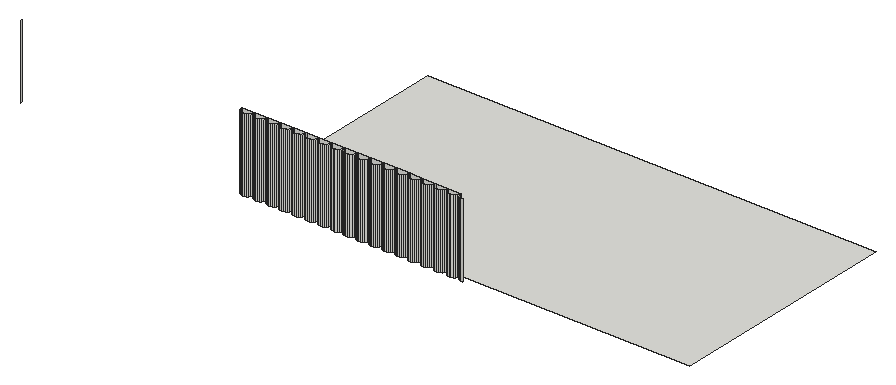
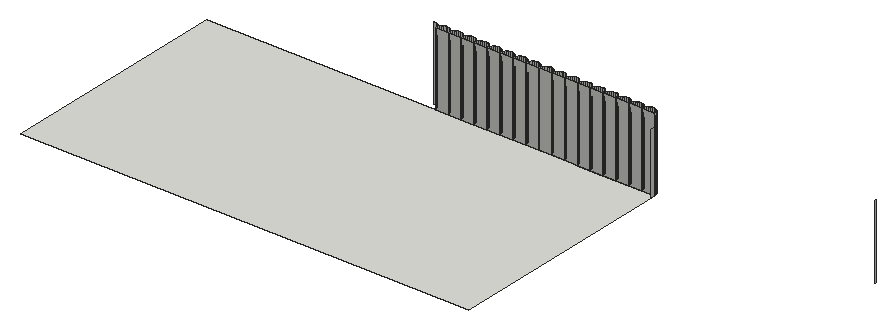
# SketchUp Ruby script. Lengths in inches.
U = 1.inch
M = Sketchup.active_model
def pt(a) = Geom::Point3d.new(a.map { |v| v * U })
def face(e, loops, mat)
  f = e.add_face(loops[0].map { |a| pt(a) })
  loops[1..].each { |l| e.add_face(l.map { |a| pt(a) }).erase! }
  f.material = f.back_material = mat if mat
  f
end
# faces: each face lists its corners as indices into pts; further lists are holes
def faces(e, pts, list, mat = nil) = list.each { |f| face(e, (f[0].is_a?(Array) ? f : [f]).map { |l| l.map { |i| pts[i] } }, mat) }
# xy, xz, yz: faces in a plane at the given z, y or x. An outline is a flat list of corners, or four numbers for a rectangle; further outlines are holes
def ring(l) = l.size == 4 ? [[l[0], l[1]], [l[2], l[1]], [l[2], l[3]], [l[0], l[3]]] : l.each_slice(2).to_a
def flat(e, list, mat, &to3) = list.each { |f| face(e, (f[0].is_a?(Array) ? f : [f]).map { |l| ring(l).map { |u, v| to3.(u, v) } }, mat) }
def xy(e, z, list, mat = nil) = flat(e, list, mat) { |x, y| [x, y, z] }
def xz(e, y, list, mat = nil) = flat(e, list, mat) { |x, z| [x, y, z] }
def yz(e, x, list, mat = nil) = flat(e, list, mat) { |y, z| [x, y, z] }
def lines(e, pts, list) = list.each { |a, b| e.add_line(pt(pts[a]), pt(pts[b])) }
# prism: a flat outline (further loops are holes) pulled along v
def prism(e, loops, v, mat = nil)
  f = face(e, loops, mat); d = Geom::Vector3d.new(v.map { |x| x * U })
  f.pushpull(f.normal.samedirection?(d) ? d.length : -d.length)
end
def box(e, o, s, mat = nil) = prism(e, [[o, [o[0] + s[0], o[1], o[2]], [o[0] + s[0], o[1] + s[1], o[2]], [o[0], o[1] + s[1], o[2]]]], [0, 0, s[2]], mat)
def at(x, y, z, deg = 0) = Geom::Transformation.translation(pt([x, y, z])) * Geom::Transformation.rotation(ORIGIN, Z_AXIS, deg.degrees)
def axes(o, x, y, z) = Geom::Transformation.new([*x, 0, *y, 0, *z, 0, *pt(o).to_a, 1])
def part(name) = M.definitions.add(name)
# library, detail: a bought-in or finely detailed component or shape, given as its bounding box
def library(name, o, s) = part(name).tap { |d| box(d.entities, o, s) }
def detail(e, o, s) = box(e.add_group.entities, o, s)
def put(e, d, t, mat = nil) = e.add_instance(d, t).tap { |i| i.material = mat if mat }
def group(e, t, mat = nil) = e.add_group.tap { |g| g.transformation = t; g.material = mat if mat }.entities
root = M.entities
xy(root,33.18,[[74.21,140.54,74.05,140.5625,73.89,140.63,73.75,140.73,73.65,140.87,73.58,141.03,73.56,141.2,74.87,141.2,74.85,141.03,74.78,140.87,74.68,140.73,74.54,140.63,74.38,140.5625],[75.53,140.54,75.36,140.5625,75.2,140.63,75.0625,140.73,74.96,140.87,74.89,141.03,74.87,141.2,76.18,141.2,76.16,141.03,76.1,140.87,75.99,140.73,75.86,140.63,75.7,140.5625],[76.84,140.54,76.67,140.5625,76.51,140.63,76.375,140.73,76.27,140.87,76.21,141.03,76.18,141.2,77.5,141.2,77.47,141.03,77.41,140.87,77.3,140.73,77.17,140.63,77.01,140.5625],[78.15,140.54,77.98,140.5625,77.82,140.63,77.6875,140.73,77.58,140.87,77.52,141.03,77.5,141.2,78.81,141.2,78.79,141.03,78.72,140.87,78.62,140.73,78.48,140.63,78.32,140.5625],[79.46,140.54,79.3,140.5625,79.14,140.63,79,140.73,78.9,140.87,78.83,141.03,78.81,141.2,80.12,141.2,80.1,141.03,80.03,140.87,79.93,140.73,79.79,140.63,79.63,140.5625],
  [80.78,140.54,80.61,140.5625,80.45,140.63,80.3125,140.73,80.21,140.87,80.14,141.03,80.12,141.2,81.43,141.2,81.41,141.03,81.35,140.87,81.24,140.73,81.11,140.63,80.95,140.5625],[82.09,140.54,81.92,140.5625,81.76,140.63,81.625,140.73,81.52,140.87,81.46,141.03,81.43,141.2,82.75,141.2,82.72,141.03,82.66,140.87,82.55,140.73,82.42,140.63,82.26,140.5625],[83.4,140.54,83.23,140.5625,83.07,140.63,82.9375,140.73,82.83,140.87,82.77,141.03,82.75,141.2,84.06,141.2,84.04,141.03,83.97,140.87,83.87,140.73,83.73,140.63,83.57,140.5625],[84.71,140.54,84.55,140.5625,84.39,140.63,84.25,140.73,84.15,140.87,84.08,141.03,84.06,141.2,85.37,141.2,85.35,141.03,85.28,140.87,85.18,140.73,85.04,140.63,84.88,140.5625],[86.03,140.54,85.86,140.5625,85.7,140.63,85.5625,140.73,85.46,140.87,85.39,141.03,85.37,141.2,86.68,141.2,86.66,141.03,86.6,140.87,86.49,140.73,86.36,140.63,86.2,140.5625],
  [87.34,140.54,87.17,140.5625,87.01,140.63,86.875,140.73,86.77,140.87,86.71,141.03,86.68,141.2,88,141.2,87.97,141.03,87.91,140.87,87.8,140.73,87.67,140.63,87.51,140.5625],[88.65,140.54,88.48,140.5625,88.32,140.63,88.1875,140.73,88.08,140.87,88.02,141.03,88,141.2,89.31,141.2,89.29,141.03,89.22,140.87,89.12,140.73,88.98,140.63,88.82,140.5625],[89.96,140.54,89.8,140.5625,89.64,140.63,89.5,140.73,89.4,140.87,89.33,141.03,89.31,141.2,90.62,141.2,90.6,141.03,90.53,140.87,90.43,140.73,90.29,140.63,90.13,140.5625],[91.28,140.54,91.11,140.5625,90.95,140.63,90.8125,140.73,90.71,140.87,90.64,141.03,90.62,141.2,91.93,141.2,91.91,141.03,91.85,140.87,91.74,140.73,91.61,140.63,91.45,140.5625],[92.59,140.54,92.42,140.5625,92.26,140.63,92.125,140.73,92.02,140.87,91.96,141.03,91.93,141.2,93.25,141.2,93.22,141.03,93.16,140.87,93.05,140.73,92.92,140.63,92.76,140.5625],
  [93.9,140.54,93.73,140.5625,93.57,140.63,93.4375,140.73,93.33,140.87,93.27,141.03,93.25,141.2,94.56,141.2,94.54,141.03,94.47,140.87,94.37,140.73,94.23,140.63,94.07,140.5625],[95.21,140.54,95.05,140.5625,94.89,140.63,94.75,140.73,94.65,140.87,94.58,141.03,94.56,141.2,95.87,141.2,95.85,141.03,95.78,140.87,95.68,140.73,95.54,140.63,95.38,140.5625],[73.56,141.2,119.1875,164.88]])
xz(root,141.2,[[73.56,33.18,74.87,40.6875],[74.87,33.18,76.18,40.6875],[76.18,33.18,77.5,40.6875],[77.5,33.18,78.81,40.6875],[78.81,33.18,80.12,40.6875],
  [80.12,33.18,81.43,40.6875],[81.43,33.18,82.75,40.6875],[82.75,33.18,84.06,40.6875],[84.06,33.18,85.37,40.6875],[85.37,33.18,86.68,40.6875],
  [86.68,33.18,88,40.6875],[88,33.18,89.31,40.6875],[89.31,33.18,90.62,40.6875],[90.62,33.18,91.93,40.6875],[91.93,33.18,93.25,40.6875],
  [93.25,33.18,94.56,40.6875],[94.56,33.18,95.87,40.6875]])
yz(root,73.56,[[141.2,33.18,141.7,39.45]])
p = [[74.05,140.5625,33.18],[74.21,140.54,33.18],[74.21,140.54,40.6875],[74.05,140.5625,40.6875],[74.38,140.5625,33.18],[74.38,140.5625,40.6875],
  [75.36,140.5625,33.18],[75.53,140.54,33.18],[75.53,140.54,40.6875],[75.36,140.5625,40.6875],[75.7,140.5625,33.18],[75.7,140.5625,40.6875],
  [76.67,140.5625,33.18],[76.84,140.54,33.18],[76.84,140.54,40.6875],[76.67,140.5625,40.6875],[77.01,140.5625,33.18],[77.01,140.5625,40.6875],
  [77.98,140.5625,33.18],[78.15,140.54,33.18],[78.15,140.54,40.6875],[77.98,140.5625,40.6875],[78.32,140.5625,33.18],[78.32,140.5625,40.6875],
  [79.3,140.5625,33.18],[79.46,140.54,33.18],[79.46,140.54,40.6875],[79.3,140.5625,40.6875],[79.63,140.5625,33.18],[79.63,140.5625,40.6875],
  [80.61,140.5625,33.18],[80.78,140.54,33.18],[80.78,140.54,40.6875],[80.61,140.5625,40.6875],[80.95,140.5625,33.18],[80.95,140.5625,40.6875],
  [81.92,140.5625,33.18],[82.09,140.54,33.18],[82.09,140.54,40.6875],[81.92,140.5625,40.6875],[82.26,140.5625,33.18],[82.26,140.5625,40.6875],
  [83.23,140.5625,33.18],[83.4,140.54,33.18],[83.4,140.54,40.6875],[83.23,140.5625,40.6875],[83.57,140.5625,33.18],[83.57,140.5625,40.6875],
  [84.55,140.5625,33.18],[84.71,140.54,33.18],[84.71,140.54,40.6875],[84.55,140.5625,40.6875],[84.88,140.5625,33.18],[84.88,140.5625,40.6875],
  [85.86,140.5625,33.18],[86.03,140.54,33.18],[86.03,140.54,40.6875],[85.86,140.5625,40.6875],[86.2,140.5625,33.18],[86.2,140.5625,40.6875],
  [87.17,140.5625,33.18],[87.34,140.54,33.18],[87.34,140.54,40.6875],[87.17,140.5625,40.6875],[87.51,140.5625,33.18],[87.51,140.5625,40.6875],
  [88.48,140.5625,33.18],[88.65,140.54,33.18],[88.65,140.54,40.6875],[88.48,140.5625,40.6875],[88.82,140.5625,33.18],[88.82,140.5625,40.6875],
  [89.8,140.5625,33.18],[89.96,140.54,33.18],[89.96,140.54,40.6875],[89.8,140.5625,40.6875],[90.13,140.5625,33.18],[90.13,140.5625,40.6875],
  [91.11,140.5625,33.18],[91.28,140.54,33.18],[91.28,140.54,40.6875],[91.11,140.5625,40.6875],[91.45,140.5625,33.18],[91.45,140.5625,40.6875],
  [92.42,140.5625,33.18],[92.59,140.54,33.18],[92.59,140.54,40.6875],[92.42,140.5625,40.6875],[92.76,140.5625,33.18],[92.76,140.5625,40.6875],
  [93.73,140.5625,33.18],[93.9,140.54,33.18],[93.9,140.54,40.6875],[93.73,140.5625,40.6875],[94.07,140.5625,33.18],[94.07,140.5625,40.6875],
  [95.05,140.5625,33.18],[95.21,140.54,33.18],[95.21,140.54,40.6875],[95.05,140.5625,40.6875],[95.38,140.5625,33.18],[95.38,140.5625,40.6875],
  [96.36,140.5625,33.18],[96.53,140.54,33.18],[96.53,140.54,40.6875],[96.36,140.5625,40.6875],[73.75,140.73,33.18],[73.89,140.63,33.18],
  [73.89,140.63,40.6875],[73.75,140.73,40.6875],[74.54,140.63,33.18],[74.54,140.63,40.6875],[74.68,140.73,33.18],[74.68,140.73,40.6875],
  [75.0625,140.73,33.18],[75.2,140.63,33.18],[75.2,140.63,40.6875],[75.0625,140.73,40.6875],[75.86,140.63,33.18],[75.86,140.63,40.6875],
  [75.99,140.73,33.18],[75.99,140.73,40.6875],[76.375,140.73,33.18],[76.51,140.63,33.18],[76.51,140.63,40.6875],[76.375,140.73,40.6875],
  [77.17,140.63,33.18],[77.17,140.63,40.6875],[77.3,140.73,33.18],[77.3,140.73,40.6875],[77.6875,140.73,33.18],[77.82,140.63,33.18],
  [77.82,140.63,40.6875],[77.6875,140.73,40.6875],[78.48,140.63,33.18],[78.48,140.63,40.6875],[78.62,140.73,33.18],[78.62,140.73,40.6875],
  [79,140.73,33.18],[79.14,140.63,33.18],[79.14,140.63,40.6875],[79,140.73,40.6875],[79.79,140.63,33.18],[79.79,140.63,40.6875],
  [79.93,140.73,33.18],[79.93,140.73,40.6875],[80.3125,140.73,33.18],[80.45,140.63,33.18],[80.45,140.63,40.6875],[80.3125,140.73,40.6875],
  [81.11,140.63,33.18],[81.11,140.63,40.6875],[81.24,140.73,33.18],[81.24,140.73,40.6875],[81.625,140.73,33.18],[81.76,140.63,33.18],
  [81.76,140.63,40.6875],[81.625,140.73,40.6875],[82.42,140.63,33.18],[82.42,140.63,40.6875],[82.55,140.73,33.18],[82.55,140.73,40.6875],
  [82.9375,140.73,33.18],[83.07,140.63,33.18],[83.07,140.63,40.6875],[82.9375,140.73,40.6875],[83.73,140.63,33.18],[83.73,140.63,40.6875],
  [83.87,140.73,33.18],[83.87,140.73,40.6875],[84.25,140.73,33.18],[84.39,140.63,33.18],[84.39,140.63,40.6875],[84.25,140.73,40.6875],
  [85.04,140.63,33.18],[85.04,140.63,40.6875],[85.18,140.73,33.18],[85.18,140.73,40.6875],[85.5625,140.73,33.18],[85.7,140.63,33.18],
  [85.7,140.63,40.6875],[85.5625,140.73,40.6875],[86.36,140.63,33.18],[86.36,140.63,40.6875],[86.49,140.73,33.18],[86.49,140.73,40.6875],
  [86.875,140.73,33.18],[87.01,140.63,33.18],[87.01,140.63,40.6875],[86.875,140.73,40.6875],[87.67,140.63,33.18],[87.67,140.63,40.6875],
  [87.8,140.73,33.18],[87.8,140.73,40.6875],[88.1875,140.73,33.18],[88.32,140.63,33.18],[88.32,140.63,40.6875],[88.1875,140.73,40.6875],
  [88.98,140.63,33.18],[88.98,140.63,40.6875],[89.12,140.73,33.18],[89.12,140.73,40.6875],[89.5,140.73,33.18],[89.64,140.63,33.18],
  [89.64,140.63,40.6875],[89.5,140.73,40.6875],[90.29,140.63,33.18],[90.29,140.63,40.6875],[90.43,140.73,33.18],[90.43,140.73,40.6875],
  [90.8125,140.73,33.18],[90.95,140.63,33.18],[90.95,140.63,40.6875],[90.8125,140.73,40.6875],[91.61,140.63,33.18],[91.61,140.63,40.6875],
  [91.74,140.73,33.18],[91.74,140.73,40.6875],[92.125,140.73,33.18],[92.26,140.63,33.18],[92.26,140.63,40.6875],[92.125,140.73,40.6875],
  [92.92,140.63,33.18],[92.92,140.63,40.6875],[93.05,140.73,33.18],[93.05,140.73,40.6875],[93.4375,140.73,33.18],[93.57,140.63,33.18],
  [93.57,140.63,40.6875],[93.4375,140.73,40.6875],[94.23,140.63,33.18],[94.23,140.63,40.6875],[94.37,140.73,33.18],[94.37,140.73,40.6875],
  [94.75,140.73,33.18],[94.89,140.63,33.18],[94.89,140.63,40.6875],[94.75,140.73,40.6875],[95.54,140.63,33.18],[95.54,140.63,40.6875],
  [95.68,140.73,33.18],[95.68,140.73,40.6875],[96.0625,140.73,33.18],[96.2,140.63,33.18],[96.2,140.63,40.6875],[96.0625,140.73,40.6875],
  [73.65,140.87,33.18],[73.65,140.87,40.6875],[74.78,140.87,33.18],[74.78,140.87,40.6875],[74.96,140.87,33.18],[74.96,140.87,40.6875],
  [76.1,140.87,33.18],[76.1,140.87,40.6875],[76.27,140.87,33.18],[76.27,140.87,40.6875],[77.41,140.87,33.18],[77.41,140.87,40.6875],
  [77.58,140.87,33.18],[77.58,140.87,40.6875],[78.72,140.87,33.18],[78.72,140.87,40.6875],[78.9,140.87,33.18],[78.9,140.87,40.6875],
  [80.03,140.87,33.18],[80.03,140.87,40.6875],[80.21,140.87,33.18],[80.21,140.87,40.6875],[81.35,140.87,33.18],[81.35,140.87,40.6875],
  [81.52,140.87,33.18],[81.52,140.87,40.6875],[82.66,140.87,33.18],[82.66,140.87,40.6875],[82.83,140.87,33.18],[82.83,140.87,40.6875],
  [83.97,140.87,33.18],[83.97,140.87,40.6875],[84.15,140.87,33.18],[84.15,140.87,40.6875],[85.28,140.87,33.18],[85.28,140.87,40.6875],
  [85.46,140.87,33.18],[85.46,140.87,40.6875],[86.6,140.87,33.18],[86.6,140.87,40.6875],[86.77,140.87,33.18],[86.77,140.87,40.6875],
  [87.91,140.87,33.18],[87.91,140.87,40.6875],[88.08,140.87,33.18],[88.08,140.87,40.6875],[89.22,140.87,33.18],[89.22,140.87,40.6875],
  [89.4,140.87,33.18],[89.4,140.87,40.6875],[90.53,140.87,33.18],[90.53,140.87,40.6875],[90.71,140.87,33.18],[90.71,140.87,40.6875],
  [91.85,140.87,33.18],[91.85,140.87,40.6875],[92.02,140.87,33.18],[92.02,140.87,40.6875],[93.16,140.87,33.18],[93.16,140.87,40.6875],
  [93.33,140.87,33.18],[93.33,140.87,40.6875],[94.47,140.87,33.18],[94.47,140.87,40.6875],[94.65,140.87,33.18],[94.65,140.87,40.6875],
  [95.78,140.87,33.18],[95.78,140.87,40.6875],[95.96,140.87,33.18],[95.96,140.87,40.6875],[73.58,141.03,33.18],[73.58,141.03,40.6875],
  [74.85,141.03,33.18],[74.85,141.03,40.6875],[74.89,141.03,33.18],[74.89,141.03,40.6875],[76.16,141.03,33.18],[76.16,141.03,40.6875],
  [76.21,141.03,33.18],[76.21,141.03,40.6875],[77.47,141.03,33.18],[77.47,141.03,40.6875],[77.52,141.03,33.18],[77.52,141.03,40.6875],
  [78.79,141.03,33.18],[78.79,141.03,40.6875],[78.83,141.03,33.18],[78.83,141.03,40.6875],[80.1,141.03,33.18],[80.1,141.03,40.6875],
  [80.14,141.03,33.18],[80.14,141.03,40.6875],[81.41,141.03,33.18],[81.41,141.03,40.6875],[81.46,141.03,33.18],[81.46,141.03,40.6875],
  [82.72,141.03,33.18],[82.72,141.03,40.6875],[82.77,141.03,33.18],[82.77,141.03,40.6875],[84.04,141.03,33.18],[84.04,141.03,40.6875],
  [84.08,141.03,33.18],[84.08,141.03,40.6875],[85.35,141.03,33.18],[85.35,141.03,40.6875],[85.39,141.03,33.18],[85.39,141.03,40.6875],
  [86.66,141.03,33.18],[86.66,141.03,40.6875],[86.71,141.03,33.18],[86.71,141.03,40.6875],[87.97,141.03,33.18],[87.97,141.03,40.6875],
  [88.02,141.03,33.18],[88.02,141.03,40.6875],[89.29,141.03,33.18],[89.29,141.03,40.6875],[89.33,141.03,33.18],[89.33,141.03,40.6875],
  [90.6,141.03,33.18],[90.6,141.03,40.6875],[90.64,141.03,33.18],[90.64,141.03,40.6875],[91.91,141.03,33.18],[91.91,141.03,40.6875],
  [91.96,141.03,33.18],[91.96,141.03,40.6875],[93.22,141.03,33.18],[93.22,141.03,40.6875],[93.27,141.03,33.18],[93.27,141.03,40.6875],
  [94.54,141.03,33.18],[94.54,141.03,40.6875],[94.58,141.03,33.18],[94.58,141.03,40.6875],[95.85,141.03,33.18],[95.85,141.03,40.6875],
  [95.89,141.03,33.18],[95.89,141.03,40.6875],[73.56,141.2,33.18],[73.56,141.2,40.6875],[73.56,141.2,39.45],[74.87,141.2,33.18],
  [74.87,141.2,40.6875],[76.18,141.2,33.18],[76.18,141.2,40.6875],[77.5,141.2,33.18],[77.5,141.2,40.6875],[78.81,141.2,33.18],
  [78.81,141.2,40.6875],[80.12,141.2,33.18],[80.12,141.2,40.6875],[81.43,141.2,33.18],[81.43,141.2,40.6875],[82.75,141.2,33.18],
  [82.75,141.2,40.6875],[84.06,141.2,33.18],[84.06,141.2,40.6875],[85.37,141.2,33.18],[85.37,141.2,40.6875],[86.68,141.2,33.18],
  [86.68,141.2,40.6875],[88,141.2,33.18],[88,141.2,40.6875],[89.31,141.2,33.18],[89.31,141.2,40.6875],[90.62,141.2,33.18],
  [90.62,141.2,40.6875],[91.93,141.2,33.18],[91.93,141.2,40.6875],[93.25,141.2,33.18],[93.25,141.2,40.6875],[94.56,141.2,33.18],
  [94.56,141.2,40.6875],[95.87,141.2,33.18],[95.87,141.2,40.6875],[51.01,141.2,33.18],[51.03,141.37,33.18],[51.03,141.37,40.6875],
  [51.01,141.2,40.6875],[51.01,141.2,39.45]]
faces(root,p,[[0,1,2,3],[1,4,5,2],[6,7,8,9],[7,10,11,8],[12,13,14,15],[13,16,17,14],[18,19,20,21],[19,22,23,20],
  [24,25,26,27],[25,28,29,26],[30,31,32,33],[31,34,35,32],[36,37,38,39],[37,40,41,38],[42,43,44,45],[43,46,47,44],
  [48,49,50,51],[49,52,53,50],[54,55,56,57],[55,58,59,56],[60,61,62,63],[61,64,65,62],[66,67,68,69],[67,70,71,68],
  [72,73,74,75],[73,76,77,74],[78,79,80,81],[79,82,83,80],[84,85,86,87],[85,88,89,86],[90,91,92,93],[91,94,95,92],
  [96,97,98,99],[97,100,101,98],[102,103,104,105],[106,107,108,109],[107,0,3,108],[4,110,111,5],[110,112,113,111],[114,115,116,117],
  [115,6,9,116],[10,118,119,11],[118,120,121,119],[122,123,124,125],[123,12,15,124],[16,126,127,17],[126,128,129,127],[130,131,132,133],
  [131,18,21,132],[22,134,135,23],[134,136,137,135],[138,139,140,141],[139,24,27,140],[28,142,143,29],[142,144,145,143],[146,147,148,149],
  [147,30,33,148],[34,150,151,35],[150,152,153,151],[154,155,156,157],[155,36,39,156],[40,158,159,41],[158,160,161,159],[162,163,164,165],
  [163,42,45,164],[46,166,167,47],[166,168,169,167],[170,171,172,173],[171,48,51,172],[52,174,175,53],[174,176,177,175],[178,179,180,181],
  [179,54,57,180],[58,182,183,59],[182,184,185,183],[186,187,188,189],[187,60,63,188],[64,190,191,65],[190,192,193,191],[194,195,196,197],
  [195,66,69,196],[70,198,199,71],[198,200,201,199],[202,203,204,205],[203,72,75,204],[76,206,207,77],[206,208,209,207],[210,211,212,213],
  [211,78,81,212],[82,214,215,83],[214,216,217,215],[218,219,220,221],[219,84,87,220],[88,222,223,89],[222,224,225,223],[226,227,228,229],
  [227,90,93,228],[94,230,231,95],[230,232,233,231],[234,235,236,237],[235,96,99,236],[100,238,239,101],[238,240,241,239],[242,243,244,245],
  [243,102,105,244],[246,106,109,247],[112,248,249,113],[250,114,117,251],[120,252,253,121],[254,122,125,255],[128,256,257,129],[258,130,133,259],
  [136,260,261,137],[262,138,141,263],[144,264,265,145],[266,146,149,267],[152,268,269,153],[270,154,157,271],[160,272,273,161],[274,162,165,275],
  [168,276,277,169],[278,170,173,279],[176,280,281,177],[282,178,181,283],[184,284,285,185],[286,186,189,287],[192,288,289,193],[290,194,197,291],
  [200,292,293,201],[294,202,205,295],[208,296,297,209],[298,210,213,299],[216,300,301,217],[302,218,221,303],[224,304,305,225],[306,226,229,307],
  [232,308,309,233],[310,234,237,311],[240,312,313,241],[314,242,245,315],[316,246,247,317],[248,318,319,249],[320,250,251,321],[252,322,323,253],
  [324,254,255,325],[256,326,327,257],[328,258,259,329],[260,330,331,261],[332,262,263,333],[264,334,335,265],[336,266,267,337],[268,338,339,269],
  [340,270,271,341],[272,342,343,273],[344,274,275,345],[276,346,347,277],[348,278,279,349],[280,350,351,281],[352,282,283,353],[284,354,355,285],
  [356,286,287,357],[288,358,359,289],[360,290,291,361],[292,362,363,293],[364,294,295,365],[296,366,367,297],[368,298,299,369],[300,370,371,301],
  [372,302,303,373],[304,374,375,305],[376,306,307,377],[308,378,379,309],[380,310,311,381],[312,382,383,313],[384,314,315,385],[386,316,317,387,388],
  [318,389,390,319],[389,320,321,390],[322,391,392,323],[391,324,325,392],[326,393,394,327],[393,328,329,394],[330,395,396,331],[395,332,333,396],
  [334,397,398,335],[397,336,337,398],[338,399,400,339],[399,340,341,400],[342,401,402,343],[401,344,345,402],[346,403,404,347],[403,348,349,404],
  [350,405,406,351],[405,352,353,406],[354,407,408,355],[407,356,357,408],[358,409,410,359],[409,360,361,410],[362,411,412,363],[411,364,365,412],
  [366,413,414,367],[413,368,369,414],[370,415,416,371],[415,372,373,416],[374,417,418,375],[417,376,377,418],[378,419,420,379],[419,380,381,420],
  [382,421,422,383],[421,384,385,422],[423,424,425,426,427]])
